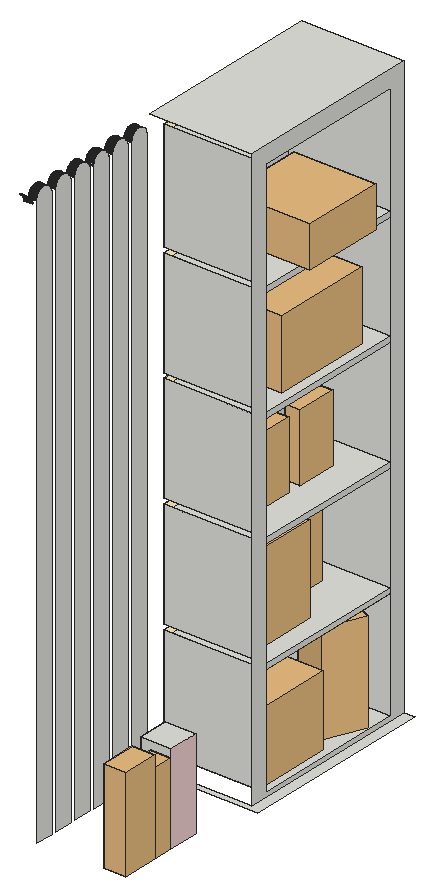
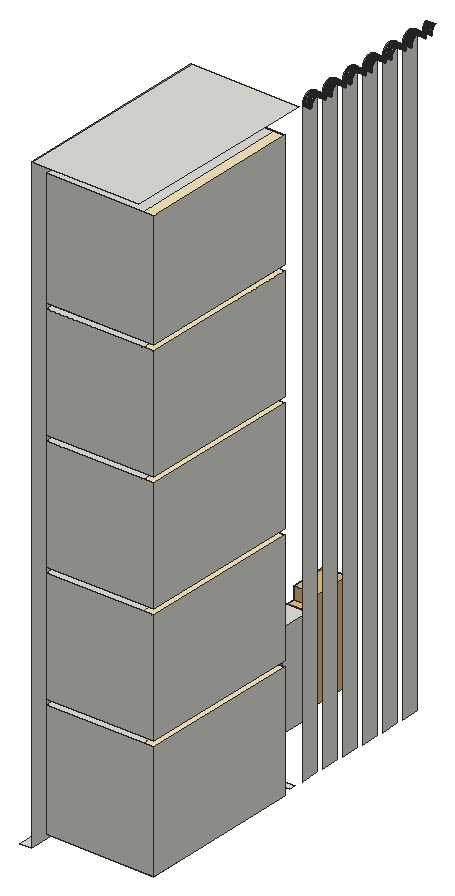
# SketchUp Ruby script. Lengths in inches.
U = 1.inch
M = Sketchup.active_model
def pt(a) = Geom::Point3d.new(a.map { |v| v * U })
def face(e, loops, mat)
  f = e.add_face(loops[0].map { |a| pt(a) })
  loops[1..].each { |l| e.add_face(l.map { |a| pt(a) }).erase! }
  f.material = f.back_material = mat if mat
  f
end
# faces: each face lists its corners as indices into pts; further lists are holes
def faces(e, pts, list, mat = nil) = list.each { |f| face(e, (f[0].is_a?(Array) ? f : [f]).map { |l| l.map { |i| pts[i] } }, mat) }
# xy, xz, yz: faces in a plane at the given z, y or x. An outline is a flat list of corners, or four numbers for a rectangle; further outlines are holes
def ring(l) = l.size == 4 ? [[l[0], l[1]], [l[2], l[1]], [l[2], l[3]], [l[0], l[3]]] : l.each_slice(2).to_a
def flat(e, list, mat, &to3) = list.each { |f| face(e, (f[0].is_a?(Array) ? f : [f]).map { |l| ring(l).map { |u, v| to3.(u, v) } }, mat) }
def xy(e, z, list, mat = nil) = flat(e, list, mat) { |x, y| [x, y, z] }
def xz(e, y, list, mat = nil) = flat(e, list, mat) { |x, z| [x, y, z] }
def yz(e, x, list, mat = nil) = flat(e, list, mat) { |y, z| [x, y, z] }
def lines(e, pts, list) = list.each { |a, b| e.add_line(pt(pts[a]), pt(pts[b])) }
# prism: a flat outline (further loops are holes) pulled along v
def prism(e, loops, v, mat = nil)
  f = face(e, loops, mat); d = Geom::Vector3d.new(v.map { |x| x * U })
  f.pushpull(f.normal.samedirection?(d) ? d.length : -d.length)
end
def box(e, o, s, mat = nil) = prism(e, [[o, [o[0] + s[0], o[1], o[2]], [o[0] + s[0], o[1] + s[1], o[2]], [o[0], o[1] + s[1], o[2]]]], [0, 0, s[2]], mat)
def at(x, y, z, deg = 0) = Geom::Transformation.translation(pt([x, y, z])) * Geom::Transformation.rotation(ORIGIN, Z_AXIS, deg.degrees)
def axes(o, x, y, z) = Geom::Transformation.new([*x, 0, *y, 0, *z, 0, *pt(o).to_a, 1])
def part(name) = M.definitions.add(name)
# library, detail: a bought-in or finely detailed component or shape, given as its bounding box
def library(name, o, s) = part(name).tap { |d| box(d.entities, o, s) }
def detail(e, o, s) = box(e.add_group.entities, o, s)
def put(e, d, t, mat = nil) = e.add_instance(d, t).tap { |i| i.material = mat if mat }
def group(e, t, mat = nil) = e.add_group.tap { |g| g.transformation = t; g.material = mat if mat }.entities
root = M.entities
M.materials.add("Heather_PantShadow").color = [249, 233, 187]
M.materials.add("Pomeli-edt-511x511").color = [242, 209, 211]
M.materials.add("profumo-muschio-natures-511x511").color = [223, 234, 229]
c1 = library("Toiletry bottle \#3",[0,0,0],[4.22,2.62,10.91])
c2 = library("Toiletry bottle \#1",[0,0,0],[3.45,3.45,11.12])
c3 = part("Component\#17")
xy(c3.entities,0,[[0,0,3.21,3.15]],"profumo-muschio-natures-511x511")
xy(c3.entities,9.32,[[0,0,3.21,3.15]])
xz(c3.entities,0,[[0,0,3.21,9.32]],"Pomeli-edt-511x511")
xz(c3.entities,3.15,[[0,0,3.21,9.32]])
yz(c3.entities,0,[[0,0,3.15,9.32]])
yz(c3.entities,3.21,[[0,0,3.15,9.32]])
c4 = library("FILE+KEEPER",[308.125,87.4375,-0.08],[14,9.09,13.53])
c5 = library("Group\#6",[0,0,0],[23.16,7,38.98])
c6 = library("Plant",[-15.17,-14.95,0],[35.27,31.45,46.14])
c7 = library("ADORNOS+-+RMLLR",[6.19,-1.3125,-0.22],[15.35,11.9,12.07])
c8 = library("Potted plant",[0.24,-1.94,0],[14.49,14.49,6.23])
c9 = library("Group\#5",[0,0,0],[23.16,7,38.98])
c10 = library("Man+sculpture",[-5.14,-9.4,0],[7.87,19.56,27.58])
c11 = library("Abstract sculpture",[0,0.06,0],[4.875,4.76,11.74])
xy(root,39.466,[[10,88.07,22.25,88.07,22.25,111,21,111,21,88.732,10,88.732]])
xy(root,40,[[9,90.732,21,109]])
xy(root,52.9,[[10.106,90.732,21,108.993],[9,108.993,21,109]])
xy(root,52.9,[[9,90.732,10.106,108.993]],"Heather_PantShadow")
xy(root,53.5,[[9,90.732,21,109]])
xy(root,66.1,[[10.106,90.732,21,108.993],[9,108.993,21,109]])
xy(root,66.1,[[9,90.732,10.106,108.993]],"Heather_PantShadow")
xy(root,66.7,[[9,90.732,21,109]])
xy(root,79.3,[[10.106,90.732,21,108.993],[9,108.993,10.106,109],[10.106,108.993,21,109]])
xy(root,79.3,[[9,90.732,10.106,108.993]],"Heather_PantShadow")
xy(root,79.9,[[9,90.732,21,109]])
xy(root,92.5,[[10.106,90.732,21,108.993],[9,108.993,10.106,109],[10.106,108.993,21,109]])
xy(root,92.5,[[9,90.732,10.106,108.993]],"Heather_PantShadow")
xy(root,93.1,[[9,90.732,21,109]])
xy(root,106,[[10.106,90.732,21,109]])
xy(root,106,[[9,90.732,10.106,109]],"Heather_PantShadow")
xy(root,108,[[9,71.967,10,72.076],[9,74.755,10,74.864],[9,77.542,10,77.651],[9,80.33,10,80.439],[9,83.117,10,83.226],
  [9,85.905,10,86.014],[9,88.732,21,111]])
xz(root,90.732,[[9,40,21,52.9],[9,53.5,21,66.1],[9,66.7,21,79.3],[9,79.9,21,92.5],[9,93.1,21,106]])
xz(root,109,[[9,40,21,52.9],[9,53.5,21,66.1],[9,66.7,21,79.3],[9,79.9,21,92.5],[9,93.1,21,106]])
yz(root,9,[[90.732,40,109,52.9],[90.732,53.5,109,66.1],[90.732,66.7,109,79.3],[90.732,79.9,109,92.5],[90.732,93.1,109,106],
  [71.967,108,72.076,108,72.022,108.001],[74.755,108,74.864,108,74.809,108.001],[77.542,108,77.651,108,77.597,108.001],[80.33,108,80.439,108,80.384,108.001],[83.117,108,83.226,108,83.172,108.001],
  [85.905,108,86.014,108,85.959,108.001]])
yz(root,10,[[70.981,39.466,73.0625,39.466,73.0625,106.961,73.061,107.015,73.057,107.069,73.05,107.123,73.04,107.177,73.027,107.23,73.012,107.282,72.993,107.334,72.973,107.384,72.949,107.433,72.923,107.481,72.895,107.528,72.864,107.572,72.831,107.616,72.795,107.657,72.758,107.697,72.718,107.734,72.677,107.769,72.633,107.803,72.589,107.834,72.542,107.862,72.494,107.888,72.445,107.911,72.395,107.932,72.343,107.95,72.291,107.966,72.238,107.979,72.185,107.989,72.131,107.996,72.076,108,71.967,108,71.913,107.996,71.859,107.989,71.805,107.979,71.752,107.966,71.7,107.95,71.649,107.932,71.598,107.911,71.549,107.888,71.501,107.862,71.455,107.834,71.41,107.803,71.367,107.769,71.325,107.734,71.286,107.697,71.248,107.657,71.213,107.616,71.18,107.572,71.149,107.528,71.12,107.481,71.094,107.433,71.071,107.384,71.05,107.334,71.032,107.282,71.016,107.23,71.004,107.177,70.994,107.123,70.987,107.069,70.982,107.015,70.981,106.961],[73.768,39.466,75.85,39.466,75.85,106.961,75.849,107.015,75.844,107.069,75.837,107.123,75.827,107.177,75.815,107.23,75.799,107.282,75.781,107.334,75.76,107.384,75.737,107.433,75.711,107.481,75.682,107.528,75.651,107.572,75.618,107.616,75.583,107.657,75.545,107.697,75.506,107.734,75.464,107.769,75.421,107.803,75.376,107.834,75.33,107.862,75.282,107.888,75.233,107.911,75.182,107.932,75.131,107.95,75.079,107.966,75.026,107.979,74.972,107.989,74.918,107.996,74.864,108,74.755,108,74.7,107.996,74.646,107.989,74.593,107.979,74.54,107.966,74.488,107.95,74.436,107.932,74.386,107.911,74.337,107.888,74.289,107.862,74.242,107.834,74.198,107.803,74.154,107.769,74.113,107.734,74.073,107.697,74.036,107.657,74,107.616,73.967,107.572,73.936,107.528,73.908,107.481,73.882,107.433,73.858,107.384,73.838,107.334,73.819,107.282,73.804,107.23,73.791,107.177,73.781,107.123,73.774,107.069,73.77,107.015,73.768,106.961],[76.556,39.466,78.637,39.466,78.637,106.961,78.636,107.015,78.632,107.069,78.625,107.123,78.615,107.177,78.602,107.23,78.587,107.282,78.568,107.334,78.548,107.384,78.524,107.433,78.498,107.481,78.47,107.528,78.439,107.572,78.406,107.616,78.37,107.657,78.333,107.697,78.293,107.734,78.252,107.769,78.208,107.803,78.164,107.834,78.117,107.862,78.069,107.888,78.02,107.911,77.97,107.932,77.918,107.95,77.866,107.966,77.813,107.979,77.76,107.989,77.706,107.996,77.651,108,77.542,108,77.488,107.996,77.434,107.989,77.38,107.979,77.327,107.966,77.275,107.95,77.224,107.932,77.173,107.911,77.124,107.888,77.076,107.862,77.03,107.834,76.985,107.803,76.942,107.769,76.9,107.734,76.861,107.697,76.823,107.657,76.788,107.616,76.755,107.572,76.724,107.528,76.695,107.481,76.669,107.433,76.646,107.384,76.625,107.334,76.607,107.282,76.591,107.23,76.579,107.177,76.569,107.123,76.562,107.069,76.557,107.015,76.556,106.961],[79.343,39.466,81.425,39.466,81.425,106.961,81.424,107.015,81.419,107.069,81.412,107.123,81.402,107.177,81.39,107.23,81.374,107.282,81.356,107.334,81.335,107.384,81.312,107.433,81.286,107.481,81.257,107.528,81.226,107.572,81.193,107.616,81.158,107.657,81.12,107.697,81.081,107.734,81.039,107.769,80.996,107.803,80.951,107.834,80.905,107.862,80.857,107.888,80.808,107.911,80.757,107.932,80.706,107.95,80.654,107.966,80.601,107.979,80.547,107.989,80.493,107.996,80.439,108,80.33,108,80.275,107.996,80.221,107.989,80.168,107.979,80.115,107.966,80.0625,107.95,80.011,107.932,79.961,107.911,79.912,107.888,79.864,107.862,79.817,107.834,79.773,107.803,79.729,107.769,79.688,107.734,79.648,107.697,79.611,107.657,79.575,107.616,79.542,107.572,79.511,107.528,79.483,107.481,79.457,107.433,79.433,107.384,79.413,107.334,79.394,107.282,79.379,107.23,79.366,107.177,79.356,107.123,79.349,107.069,79.345,107.015,79.343,106.961],[82.131,39.466,84.212,39.466,84.212,106.961,84.211,107.015,84.207,107.069,84.2,107.123,84.19,107.177,84.177,107.23,84.162,107.282,84.143,107.334,84.123,107.384,84.099,107.433,84.073,107.481,84.045,107.528,84.014,107.572,83.981,107.616,83.945,107.657,83.908,107.697,83.868,107.734,83.827,107.769,83.783,107.803,83.739,107.834,83.692,107.862,83.644,107.888,83.595,107.911,83.545,107.932,83.493,107.95,83.441,107.966,83.388,107.979,83.335,107.989,83.281,107.996,83.226,108,83.117,108,83.063,107.996,83.009,107.989,82.955,107.979,82.902,107.966,82.85,107.95,82.799,107.932,82.748,107.911,82.699,107.888,82.651,107.862,82.605,107.834,82.56,107.803,82.517,107.769,82.475,107.734,82.436,107.697,82.398,107.657,82.363,107.616,82.33,107.572,82.299,107.528,82.27,107.481,82.244,107.433,82.221,107.384,82.2,107.334,82.182,107.282,82.166,107.23,82.154,107.177,82.144,107.123,82.137,107.069,82.132,107.015,82.131,106.961],
  [84.918,39.466,87,39.466,87,106.961,86.999,107.015,86.994,107.069,86.987,107.123,86.977,107.177,86.965,107.23,86.949,107.282,86.931,107.334,86.91,107.384,86.887,107.433,86.861,107.481,86.832,107.528,86.801,107.572,86.768,107.616,86.733,107.657,86.695,107.697,86.656,107.734,86.614,107.769,86.571,107.803,86.526,107.834,86.48,107.862,86.432,107.888,86.383,107.911,86.332,107.932,86.281,107.95,86.229,107.966,86.176,107.979,86.122,107.989,86.068,107.996,86.014,108,85.905,108,85.85,107.996,85.796,107.989,85.743,107.979,85.69,107.966,85.638,107.95,85.586,107.932,85.536,107.911,85.487,107.888,85.439,107.862,85.392,107.834,85.348,107.803,85.304,107.769,85.263,107.734,85.223,107.697,85.186,107.657,85.15,107.616,85.117,107.572,85.086,107.528,85.058,107.481,85.032,107.433,85.008,107.384,84.988,107.334,84.969,107.282,84.954,107.23,84.941,107.177,84.931,107.123,84.924,107.069,84.92,107.015,84.918,106.961]])
yz(root,21,[[[88.732,39.466,111,108],[90.732,40,109,106]],[90.732,52.9,109,53.5],[90.732,66.1,109,66.7],[90.732,79.3,109,79.9],[90.732,92.5,109,93.1]])
p = [[9,70.274,107.015],[9,70.269,107.069],[10,70.269,107.069],[10,70.274,107.015],[9,70.275,106.961],[10,70.275,106.961],
  [9,70.982,107.015],[9,70.981,106.961],[10,70.981,106.961],[10,70.982,107.015],[9,70.987,107.069],[10,70.987,107.069],
  [9,73.061,107.015],[9,73.057,107.069],[10,73.057,107.069],[10,73.061,107.015],[9,73.0625,106.961],[10,73.0625,106.961],
  [9,73.77,107.015],[9,73.768,106.961],[10,73.768,106.961],[10,73.77,107.015],[9,73.774,107.069],[10,73.774,107.069],
  [9,75.849,107.015],[9,75.844,107.069],[10,75.844,107.069],[10,75.849,107.015],[9,75.85,106.961],[10,75.85,106.961],
  [9,76.557,107.015],[9,76.556,106.961],[10,76.556,106.961],[10,76.557,107.015],[9,76.562,107.069],[10,76.562,107.069],
  [9,78.636,107.015],[9,78.632,107.069],[10,78.632,107.069],[10,78.636,107.015],[9,78.637,106.961],[10,78.637,106.961],
  [9,79.345,107.015],[9,79.343,106.961],[10,79.343,106.961],[10,79.345,107.015],[9,79.349,107.069],[10,79.349,107.069],
  [9,81.424,107.015],[9,81.419,107.069],[10,81.419,107.069],[10,81.424,107.015],[9,81.425,106.961],[10,81.425,106.961],
  [9,82.132,107.015],[9,82.131,106.961],[10,82.131,106.961],[10,82.132,107.015],[9,82.137,107.069],[10,82.137,107.069],
  [9,84.211,107.015],[9,84.207,107.069],[10,84.207,107.069],[10,84.211,107.015],[9,84.212,106.961],[10,84.212,106.961],
  [9,84.92,107.015],[9,84.918,106.961],[10,84.918,106.961],[10,84.92,107.015],[9,84.924,107.069],[10,84.924,107.069],
  [9,86.999,107.015],[9,86.994,107.069],[10,86.994,107.069],[10,86.999,107.015],[9,87,106.961],[10,87,106.961],
  [9,70.262,107.123],[9,70.252,107.177],[10,70.252,107.177],[10,70.262,107.123],[9,70.994,107.123],[10,70.994,107.123],
  [9,71.004,107.177],[10,71.004,107.177],[9,73.05,107.123],[9,73.04,107.177],[10,73.04,107.177],[10,73.05,107.123],
  [9,73.781,107.123],[10,73.781,107.123],[9,73.791,107.177],[10,73.791,107.177],[9,75.837,107.123],[9,75.827,107.177],
  [10,75.827,107.177],[10,75.837,107.123],[9,76.569,107.123],[10,76.569,107.123],[9,76.579,107.177],[10,76.579,107.177],
  [9,78.625,107.123],[9,78.615,107.177],[10,78.615,107.177],[10,78.625,107.123],[9,79.356,107.123],[10,79.356,107.123],
  [9,79.366,107.177],[10,79.366,107.177],[9,81.412,107.123],[9,81.402,107.177],[10,81.402,107.177],[10,81.412,107.123],
  [9,82.144,107.123],[10,82.144,107.123],[9,82.154,107.177],[10,82.154,107.177],[9,84.2,107.123],[9,84.19,107.177],
  [10,84.19,107.177],[10,84.2,107.123],[9,84.931,107.123],[10,84.931,107.123],[9,84.941,107.177],[10,84.941,107.177],
  [9,86.987,107.123],[9,86.977,107.177],[10,86.977,107.177],[10,86.987,107.123],[9,70.24,107.23],[9,70.224,107.282],
  [10,70.224,107.282],[10,70.24,107.23],[9,71.016,107.23],[10,71.016,107.23],[9,71.032,107.282],[10,71.032,107.282],
  [9,73.027,107.23],[9,73.012,107.282],[10,73.012,107.282],[10,73.027,107.23],[9,73.804,107.23],[10,73.804,107.23],
  [9,73.819,107.282],[10,73.819,107.282],[9,75.815,107.23],[9,75.799,107.282],[10,75.799,107.282],[10,75.815,107.23],
  [9,76.591,107.23],[10,76.591,107.23],[9,76.607,107.282],[10,76.607,107.282],[9,78.602,107.23],[9,78.587,107.282],
  [10,78.587,107.282],[10,78.602,107.23],[9,79.379,107.23],[10,79.379,107.23],[9,79.394,107.282],[10,79.394,107.282],
  [9,81.39,107.23],[9,81.374,107.282],[10,81.374,107.282],[10,81.39,107.23],[9,82.166,107.23],[10,82.166,107.23],
  [9,82.182,107.282],[10,82.182,107.282],[9,84.177,107.23],[9,84.162,107.282],[10,84.162,107.282],[10,84.177,107.23],
  [9,84.954,107.23],[10,84.954,107.23],[9,84.969,107.282],[10,84.969,107.282],[9,86.965,107.23],[9,86.949,107.282],
  [10,86.949,107.282],[10,86.965,107.23],[9,70.206,107.334],[9,70.185,107.384],[10,70.185,107.384],[10,70.206,107.334],
  [9,71.05,107.334],[10,71.05,107.334],[9,71.071,107.384],[10,71.071,107.384],[9,72.993,107.334],[9,72.973,107.384],
  [10,72.973,107.384],[10,72.993,107.334],[9,73.838,107.334],[10,73.838,107.334],[9,73.858,107.384],[10,73.858,107.384],
  [9,75.781,107.334],[9,75.76,107.384],[10,75.76,107.384],[10,75.781,107.334],[9,76.625,107.334],[10,76.625,107.334],
  [9,76.646,107.384],[10,76.646,107.384],[9,78.568,107.334],[9,78.548,107.384],[10,78.548,107.384],[10,78.568,107.334],
  [9,79.413,107.334],[10,79.413,107.334],[9,79.433,107.384],[10,79.433,107.384],[9,81.356,107.334],[9,81.335,107.384],
  [10,81.335,107.384],[10,81.356,107.334],[9,82.2,107.334],[10,82.2,107.334],[9,82.221,107.384],[10,82.221,107.384],
  [9,84.143,107.334],[9,84.123,107.384],[10,84.123,107.384],[10,84.143,107.334],[9,84.988,107.334],[10,84.988,107.334],
  [9,85.008,107.384],[10,85.008,107.384],[9,86.931,107.334],[9,86.91,107.384],[10,86.91,107.384],[10,86.931,107.334],
  [9,70.162,107.433],[9,70.136,107.481],[10,70.136,107.481],[10,70.162,107.433],[9,71.094,107.433],[10,71.094,107.433],
  [9,71.12,107.481],[10,71.12,107.481],[9,72.949,107.433],[9,72.923,107.481],[10,72.923,107.481],[10,72.949,107.433],
  [9,73.882,107.433],[10,73.882,107.433],[9,73.908,107.481],[10,73.908,107.481],[9,75.737,107.433],[9,75.711,107.481],
  [10,75.711,107.481],[10,75.737,107.433],[9,76.669,107.433],[10,76.669,107.433],[9,76.695,107.481],[10,76.695,107.481],
  [9,78.524,107.433],[9,78.498,107.481],[10,78.498,107.481],[10,78.524,107.433],[9,79.457,107.433],[10,79.457,107.433],
  [9,79.483,107.481],[10,79.483,107.481],[9,81.312,107.433],[9,81.286,107.481],[10,81.286,107.481],[10,81.312,107.433],
  [9,82.244,107.433],[10,82.244,107.433],[9,82.27,107.481],[10,82.27,107.481],[9,84.099,107.433],[9,84.073,107.481],
  [10,84.073,107.481],[10,84.099,107.433],[9,85.032,107.433],[10,85.032,107.433],[9,85.058,107.481],[10,85.058,107.481],
  [9,86.887,107.433],[9,86.861,107.481],[10,86.861,107.481],[10,86.887,107.433],[9,70.107,107.528],[9,70.076,107.572],
  [10,70.076,107.572],[10,70.107,107.528],[9,71.149,107.528],[10,71.149,107.528],[9,71.18,107.572],[10,71.18,107.572],
  [9,72.895,107.528],[9,72.864,107.572],[10,72.864,107.572],[10,72.895,107.528],[9,73.936,107.528],[10,73.936,107.528],
  [9,73.967,107.572],[10,73.967,107.572],[9,75.682,107.528],[9,75.651,107.572],[10,75.651,107.572],[10,75.682,107.528],
  [9,76.724,107.528],[10,76.724,107.528],[9,76.755,107.572],[10,76.755,107.572],[9,78.47,107.528],[9,78.439,107.572],
  [10,78.439,107.572],[10,78.47,107.528],[9,79.511,107.528],[10,79.511,107.528],[9,79.542,107.572],[10,79.542,107.572],
  [9,81.257,107.528],[9,81.226,107.572],[10,81.226,107.572],[10,81.257,107.528],[9,82.299,107.528],[10,82.299,107.528],
  [9,82.33,107.572],[10,82.33,107.572],[9,84.045,107.528],[9,84.014,107.572],[10,84.014,107.572],[10,84.045,107.528],
  [9,85.086,107.528],[10,85.086,107.528],[9,85.117,107.572],[10,85.117,107.572],[9,86.832,107.528],[9,86.801,107.572],
  [10,86.801,107.572],[10,86.832,107.528],[9,70.043,107.616],[9,70.008,107.657],[10,70.008,107.657],[10,70.043,107.616],
  [9,71.213,107.616],[10,71.213,107.616],[9,71.248,107.657],[10,71.248,107.657],[9,72.831,107.616],[9,72.795,107.657],
  [10,72.795,107.657],[10,72.831,107.616],[9,74,107.616],[10,74,107.616],[9,74.036,107.657],[10,74.036,107.657],
  [9,75.618,107.616],[9,75.583,107.657],[10,75.583,107.657],[10,75.618,107.616],[9,76.788,107.616],[10,76.788,107.616],
  [9,76.823,107.657],[10,76.823,107.657],[9,78.406,107.616],[9,78.37,107.657],[10,78.37,107.657],[10,78.406,107.616],
  [9,79.575,107.616],[10,79.575,107.616],[9,79.611,107.657],[10,79.611,107.657],[9,81.193,107.616],[9,81.158,107.657],
  [10,81.158,107.657],[10,81.193,107.616],[9,82.363,107.616],[10,82.363,107.616],[9,82.398,107.657],[10,82.398,107.657],
  [9,83.981,107.616],[9,83.945,107.657],[10,83.945,107.657],[10,83.981,107.616],[9,85.15,107.616],[10,85.15,107.616],
  [9,85.186,107.657],[10,85.186,107.657],[9,86.768,107.616],[9,86.733,107.657],[10,86.733,107.657],[10,86.768,107.616],
  [9,69.931,107.734],[9,69.889,107.769],[10,69.889,107.769],[10,69.931,107.734],[9,69.97,107.697],[10,69.97,107.697],
  [9,71.286,107.697],[10,71.286,107.697],[9,71.325,107.734],[10,71.325,107.734],[9,71.367,107.769],[10,71.367,107.769],
  [9,72.718,107.734],[9,72.677,107.769],[10,72.677,107.769],[10,72.718,107.734],[9,72.758,107.697],[10,72.758,107.697],
  [9,74.073,107.697],[10,74.073,107.697],[9,74.113,107.734],[10,74.113,107.734],[9,74.154,107.769],[10,74.154,107.769],
  [9,75.506,107.734],[9,75.464,107.769],[10,75.464,107.769],[10,75.506,107.734],[9,75.545,107.697],[10,75.545,107.697],
  [9,76.861,107.697],[10,76.861,107.697],[9,76.9,107.734],[10,76.9,107.734],[9,76.942,107.769],[10,76.942,107.769],
  [9,78.293,107.734],[9,78.252,107.769],[10,78.252,107.769],[10,78.293,107.734],[9,78.333,107.697],[10,78.333,107.697],
  [9,79.648,107.697],[10,79.648,107.697],[9,79.688,107.734],[10,79.688,107.734],[9,79.729,107.769],[10,79.729,107.769],
  [9,81.081,107.734],[9,81.039,107.769],[10,81.039,107.769],[10,81.081,107.734],[9,81.12,107.697],[10,81.12,107.697],
  [9,82.436,107.697],[10,82.436,107.697],[9,82.475,107.734],[10,82.475,107.734],[9,82.517,107.769],[10,82.517,107.769],
  [9,83.868,107.734],[9,83.827,107.769],[10,83.827,107.769],[10,83.868,107.734],[9,83.908,107.697],[10,83.908,107.697],
  [9,85.223,107.697],[10,85.223,107.697],[9,85.263,107.734],[10,85.263,107.734],[9,85.304,107.769],[10,85.304,107.769],
  [9,86.656,107.734],[9,86.614,107.769],[10,86.614,107.769],[10,86.656,107.734],[9,86.695,107.697],[10,86.695,107.697],
  [9,69.801,107.834],[9,69.755,107.862],[10,69.755,107.862],[10,69.801,107.834],[9,69.846,107.803],[10,69.846,107.803],
  [9,71.41,107.803],[10,71.41,107.803],[9,71.455,107.834],[10,71.455,107.834],[9,71.501,107.862],[10,71.501,107.862],
  [9,72.589,107.834],[9,72.542,107.862],[10,72.542,107.862],[10,72.589,107.834],[9,72.633,107.803],[10,72.633,107.803],
  [9,74.198,107.803],[10,74.198,107.803],[9,74.242,107.834],[10,74.242,107.834],[9,74.289,107.862],[10,74.289,107.862],
  [9,75.376,107.834],[9,75.33,107.862],[10,75.33,107.862],[10,75.376,107.834],[9,75.421,107.803],[10,75.421,107.803],
  [9,76.985,107.803],[10,76.985,107.803],[9,77.03,107.834],[10,77.03,107.834],[9,77.076,107.862],[10,77.076,107.862],
  [9,78.164,107.834],[9,78.117,107.862],[10,78.117,107.862],[10,78.164,107.834],[9,78.208,107.803],[10,78.208,107.803],
  [9,79.773,107.803],[10,79.773,107.803],[9,79.817,107.834],[10,79.817,107.834],[9,79.864,107.862],[10,79.864,107.862],
  [9,80.951,107.834],[9,80.905,107.862],[10,80.905,107.862],[10,80.951,107.834],[9,80.996,107.803],[10,80.996,107.803],
  [9,82.56,107.803],[10,82.56,107.803],[9,82.605,107.834],[10,82.605,107.834],[9,82.651,107.862],[10,82.651,107.862],
  [9,83.739,107.834],[9,83.692,107.862],[10,83.692,107.862],[10,83.739,107.834],[9,83.783,107.803],[10,83.783,107.803],
  [9,85.348,107.803],[10,85.348,107.803],[9,85.392,107.834],[10,85.392,107.834],[9,85.439,107.862],[10,85.439,107.862],
  [9,86.526,107.834],[9,86.48,107.862],[10,86.48,107.862],[10,86.526,107.834],[9,86.571,107.803],[10,86.571,107.803],
  [9,69.707,107.888],[10,69.707,107.888],[9,71.549,107.888],[10,71.549,107.888],[9,71.598,107.911],[10,71.598,107.911],
  [9,71.649,107.932],[10,71.649,107.932],[9,71.7,107.95],[10,71.7,107.95],[9,72.395,107.932],[9,72.343,107.95],
  [10,72.343,107.95],[10,72.395,107.932],[9,72.445,107.911],[10,72.445,107.911],[9,72.494,107.888],[10,72.494,107.888],
  [9,74.337,107.888],[10,74.337,107.888],[9,74.386,107.911],[10,74.386,107.911],[9,74.436,107.932],[10,74.436,107.932],
  [9,74.488,107.95],[10,74.488,107.95],[9,75.182,107.932],[9,75.131,107.95],[10,75.131,107.95],[10,75.182,107.932],
  [9,75.233,107.911],[10,75.233,107.911],[9,75.282,107.888],[10,75.282,107.888],[9,77.124,107.888],[10,77.124,107.888],
  [9,77.173,107.911],[10,77.173,107.911],[9,77.224,107.932],[10,77.224,107.932],[9,77.275,107.95],[10,77.275,107.95],
  [9,77.97,107.932],[9,77.918,107.95],[10,77.918,107.95],[10,77.97,107.932],[9,78.02,107.911],[10,78.02,107.911],
  [9,78.069,107.888],[10,78.069,107.888],[9,79.912,107.888],[10,79.912,107.888],[9,79.961,107.911],[10,79.961,107.911],
  [9,80.011,107.932],[10,80.011,107.932],[9,80.0625,107.95],[10,80.0625,107.95],[9,80.757,107.932],[9,80.706,107.95],
  [10,80.706,107.95],[10,80.757,107.932],[9,80.808,107.911],[10,80.808,107.911],[9,80.857,107.888],[10,80.857,107.888],
  [9,82.699,107.888],[10,82.699,107.888],[9,82.748,107.911],[10,82.748,107.911],[9,82.799,107.932],[10,82.799,107.932],
  [9,82.85,107.95],[10,82.85,107.95],[9,83.545,107.932],[9,83.493,107.95],[10,83.493,107.95],[10,83.545,107.932],
  [9,83.595,107.911],[10,83.595,107.911],[9,83.644,107.888],[10,83.644,107.888],[9,85.487,107.888],[10,85.487,107.888],
  [9,85.536,107.911],[10,85.536,107.911],[9,85.586,107.932],[10,85.586,107.932],[9,85.638,107.95],[10,85.638,107.95],
  [9,86.332,107.932],[9,86.281,107.95],[10,86.281,107.95],[10,86.332,107.932],[9,86.383,107.911],[10,86.383,107.911],
  [9,86.432,107.888],[10,86.432,107.888],[9,71.752,107.966],[10,71.752,107.966],[9,71.805,107.979],[10,71.805,107.979],
  [9,71.859,107.989],[10,71.859,107.989],[9,71.913,107.996],[10,71.913,107.996],[9,71.967,108],[10,71.967,108],
  [9,72.131,107.996],[9,72.076,108],[10,72.076,108],[10,72.131,107.996],[9,72.185,107.989],[10,72.185,107.989],
  [9,72.238,107.979],[10,72.238,107.979],[9,72.291,107.966],[10,72.291,107.966],[9,74.54,107.966],[10,74.54,107.966],
  [9,74.593,107.979],[10,74.593,107.979],[9,74.646,107.989],[10,74.646,107.989],[9,74.7,107.996],[10,74.7,107.996],
  [9,74.755,108],[10,74.755,108],[9,74.918,107.996],[9,74.864,108],[10,74.864,108],[10,74.918,107.996],
  [9,74.972,107.989],[10,74.972,107.989],[9,75.026,107.979],[10,75.026,107.979],[9,75.079,107.966],[10,75.079,107.966],
  [9,77.327,107.966],[10,77.327,107.966],[9,77.38,107.979],[10,77.38,107.979],[9,77.434,107.989],[10,77.434,107.989],
  [9,77.488,107.996],[10,77.488,107.996],[9,77.542,108],[10,77.542,108],[9,77.706,107.996],[9,77.651,108],
  [10,77.651,108],[10,77.706,107.996],[9,77.76,107.989],[10,77.76,107.989],[9,77.813,107.979],[10,77.813,107.979],
  [9,77.866,107.966],[10,77.866,107.966],[9,80.115,107.966],[10,80.115,107.966],[9,80.168,107.979],[10,80.168,107.979],
  [9,80.221,107.989],[10,80.221,107.989],[9,80.275,107.996],[10,80.275,107.996],[9,80.33,108],[10,80.33,108],
  [9,80.493,107.996],[9,80.439,108],[10,80.439,108],[10,80.493,107.996],[9,80.547,107.989],[10,80.547,107.989],
  [9,80.601,107.979],[10,80.601,107.979],[9,80.654,107.966],[10,80.654,107.966],[9,82.902,107.966],[10,82.902,107.966],
  [9,82.955,107.979],[10,82.955,107.979],[9,83.009,107.989],[10,83.009,107.989],[9,83.063,107.996],[10,83.063,107.996],
  [9,83.117,108],[10,83.117,108],[9,83.281,107.996],[9,83.226,108],[10,83.226,108],[10,83.281,107.996],
  [9,83.335,107.989],[10,83.335,107.989],[9,83.388,107.979],[10,83.388,107.979],[9,83.441,107.966],[10,83.441,107.966],
  [9,85.69,107.966],[10,85.69,107.966],[9,85.743,107.979],[10,85.743,107.979],[9,85.796,107.989],[10,85.796,107.989],
  [9,85.85,107.996],[10,85.85,107.996],[9,85.905,108],[10,85.905,108],[9,86.068,107.996],[9,86.014,108],
  [10,86.014,108],[10,86.068,107.996],[9,86.122,107.989],[10,86.122,107.989],[9,86.176,107.979],[10,86.176,107.979],
  [9,86.229,107.966],[10,86.229,107.966],[9,90.725,52.9],[9,90.732,52.9],[9,90.725,92.5],[9,90.732,92.5],
  [9,90.725,66.1],[9,90.732,66.1],[9,90.725,79.3],[9,90.732,79.3]]
faces(root,p,[[0,1,2,3],[4,0,3,5],[6,7,8,9],[10,6,9,11],[12,13,14,15],[16,12,15,17],[18,19,20,21],[22,18,21,23],
  [24,25,26,27],[28,24,27,29],[30,31,32,33],[34,30,33,35],[36,37,38,39],[40,36,39,41],[42,43,44,45],[46,42,45,47],
  [48,49,50,51],[52,48,51,53],[54,55,56,57],[58,54,57,59],[60,61,62,63],[64,60,63,65],[66,67,68,69],[70,66,69,71],
  [72,73,74,75],[76,72,75,77],[78,79,80,81],[1,78,81,2],[82,10,11,83],[84,82,83,85],[86,87,88,89],[13,86,89,14],
  [90,22,23,91],[92,90,91,93],[94,95,96,97],[25,94,97,26],[98,34,35,99],[100,98,99,101],[102,103,104,105],[37,102,105,38],
  [106,46,47,107],[108,106,107,109],[110,111,112,113],[49,110,113,50],[114,58,59,115],[116,114,115,117],[118,119,120,121],[61,118,121,62],
  [122,70,71,123],[124,122,123,125],[126,127,128,129],[73,126,129,74],[130,131,132,133],[79,130,133,80],[134,84,85,135],[136,134,135,137],
  [138,139,140,141],[87,138,141,88],[142,92,93,143],[144,142,143,145],[146,147,148,149],[95,146,149,96],[150,100,101,151],[152,150,151,153],
  [154,155,156,157],[103,154,157,104],[158,108,109,159],[160,158,159,161],[162,163,164,165],[111,162,165,112],[166,116,117,167],[168,166,167,169],
  [170,171,172,173],[119,170,173,120],[174,124,125,175],[176,174,175,177],[178,179,180,181],[127,178,181,128],[182,183,184,185],[131,182,185,132],
  [186,136,137,187],[188,186,187,189],[190,191,192,193],[139,190,193,140],[194,144,145,195],[196,194,195,197],[198,199,200,201],[147,198,201,148],
  [202,152,153,203],[204,202,203,205],[206,207,208,209],[155,206,209,156],[210,160,161,211],[212,210,211,213],[214,215,216,217],[163,214,217,164],
  [218,168,169,219],[220,218,219,221],[222,223,224,225],[171,222,225,172],[226,176,177,227],[228,226,227,229],[230,231,232,233],[179,230,233,180],
  [234,235,236,237],[183,234,237,184],[238,188,189,239],[240,238,239,241],[242,243,244,245],[191,242,245,192],[246,196,197,247],[248,246,247,249],
  [250,251,252,253],[199,250,253,200],[254,204,205,255],[256,254,255,257],[258,259,260,261],[207,258,261,208],[262,212,213,263],[264,262,263,265],
  [266,267,268,269],[215,266,269,216],[270,220,221,271],[272,270,271,273],[274,275,276,277],[223,274,277,224],[278,228,229,279],[280,278,279,281],
  [282,283,284,285],[231,282,285,232],[286,287,288,289],[235,286,289,236],[290,240,241,291],[292,290,291,293],[294,295,296,297],[243,294,297,244],
  [298,248,249,299],[300,298,299,301],[302,303,304,305],[251,302,305,252],[306,256,257,307],[308,306,307,309],[310,311,312,313],[259,310,313,260],
  [314,264,265,315],[316,314,315,317],[318,319,320,321],[267,318,321,268],[322,272,273,323],[324,322,323,325],[326,327,328,329],[275,326,329,276],
  [330,280,281,331],[332,330,331,333],[334,335,336,337],[283,334,337,284],[338,339,340,341],[287,338,341,288],[342,292,293,343],[344,342,343,345],
  [346,347,348,349],[295,346,349,296],[350,300,301,351],[352,350,351,353],[354,355,356,357],[303,354,357,304],[358,308,309,359],[360,358,359,361],
  [362,363,364,365],[311,362,365,312],[366,316,317,367],[368,366,367,369],[370,371,372,373],[319,370,373,320],[374,324,325,375],[376,374,375,377],
  [378,379,380,381],[327,378,381,328],[382,332,333,383],[384,382,383,385],[386,387,388,389],[335,386,389,336],[390,391,392,393],[394,390,393,395],
  [339,394,395,340],[396,344,345,397],[398,396,397,399],[400,398,399,401],[402,403,404,405],[406,402,405,407],[347,406,407,348],[408,352,353,409],
  [410,408,409,411],[412,410,411,413],[414,415,416,417],[418,414,417,419],[355,418,419,356],[420,360,361,421],[422,420,421,423],[424,422,423,425],
  [426,427,428,429],[430,426,429,431],[363,430,431,364],[432,368,369,433],[434,432,433,435],[436,434,435,437],[438,439,440,441],[442,438,441,443],
  [371,442,443,372],[444,376,377,445],[446,444,445,447],[448,446,447,449],[450,451,452,453],[454,450,453,455],[379,454,455,380],[456,384,385,457],
  [458,456,457,459],[460,458,459,461],[462,463,464,465],[466,462,465,467],[387,466,467,388],[468,469,470,471],[472,468,471,473],[391,472,473,392],
  [474,400,401,475],[476,474,475,477],[478,476,477,479],[480,481,482,483],[484,480,483,485],[403,484,485,404],[486,412,413,487],[488,486,487,489],
  [490,488,489,491],[492,493,494,495],[496,492,495,497],[415,496,497,416],[498,424,425,499],[500,498,499,501],[502,500,501,503],[504,505,506,507],
  [508,504,507,509],[427,508,509,428],[510,436,437,511],[512,510,511,513],[514,512,513,515],[516,517,518,519],[520,516,519,521],[439,520,521,440],
  [522,448,449,523],[524,522,523,525],[526,524,525,527],[528,529,530,531],[532,528,531,533],[451,532,533,452],[534,460,461,535],[536,534,535,537],
  [538,536,537,539],[540,541,542,543],[544,540,543,545],[463,544,545,464],[469,546,547,470],[548,478,479,549],[550,548,549,551],[552,550,551,553],
  [554,552,553,555],[556,557,558,559],[560,556,559,561],[562,560,561,563],[481,562,563,482],[564,490,491,565],[566,564,565,567],[568,566,567,569],
  [570,568,569,571],[572,573,574,575],[576,572,575,577],[578,576,577,579],[493,578,579,494],[580,502,503,581],[582,580,581,583],[584,582,583,585],
  [586,584,585,587],[588,589,590,591],[592,588,591,593],[594,592,593,595],[505,594,595,506],[596,514,515,597],[598,596,597,599],[600,598,599,601],
  [602,600,601,603],[604,605,606,607],[608,604,607,609],[610,608,609,611],[517,610,611,518],[612,526,527,613],[614,612,613,615],[616,614,615,617],
  [618,616,617,619],[620,621,622,623],[624,620,623,625],[626,624,625,627],[529,626,627,530],[628,538,539,629],[630,628,629,631],[632,630,631,633],
  [634,632,633,635],[636,637,638,639],[640,636,639,641],[642,640,641,643],[541,642,643,542],[644,554,555,645],[646,644,645,647],[648,646,647,649],
  [650,648,649,651],[652,650,651,653],[654,655,656,657],[658,654,657,659],[660,658,659,661],[662,660,661,663],[557,662,663,558],[664,570,571,665],
  [666,664,665,667],[668,666,667,669],[670,668,669,671],[672,670,671,673],[674,675,676,677],[678,674,677,679],[680,678,679,681],[682,680,681,683],
  [573,682,683,574],[684,586,587,685],[686,684,685,687],[688,686,687,689],[690,688,689,691],[692,690,691,693],[694,695,696,697],[698,694,697,699],
  [700,698,699,701],[702,700,701,703],[589,702,703,590],[704,602,603,705],[706,704,705,707],[708,706,707,709],[710,708,709,711],[712,710,711,713],
  [714,715,716,717],[718,714,717,719],[720,718,719,721],[722,720,721,723],[605,722,723,606],[724,618,619,725],[726,724,725,727],[728,726,727,729],
  [730,728,729,731],[732,730,731,733],[734,735,736,737],[738,734,737,739],[740,738,739,741],[742,740,741,743],[621,742,743,622],[744,634,635,745],
  [746,744,745,747],[748,746,747,749],[750,748,749,751],[752,750,751,753],[754,755,756,757],[758,754,757,759],[760,758,759,761],[762,760,761,763],
  [637,762,763,638]])
lines(root,p,[[764,765],[766,767],[768,769],[770,771]])
put(root,c1,at(20.1875,71.22,39.47,90))
put(root,c2,axes([20.1875,75.4375,39.47],[0,0.69,0],[-0.69,0,0],[0,0,0.85643]))
put(root,c3,axes([20.1875,77.82,39.47],[0,1.13,0],[-1.13,0,0],[0,0,1.13]))
put(root,c4,axes([-39.39,290.18,40.01],[0,-0.61622,0],[0.61622,0,0],[0,0,0.61622]))
put(root,c5,axes([17.25,94.01,66.57],[0,0.20584,0],[-0.25731,0,0],[0,0,0.20584]))
put(root,c6,axes([14.3,96.27,53.5],[0.22445,0,0],[0,0.22445,0],[0,0,0.22445]))
put(root,c7,axes([19.38,89.3,80.39],[0,0.76608,0],[-0.672,0,0],[0,0,0.672]))
put(root,c8,axes([12.39,97.06,93.1],[0.66461,0,0],[0,0.66461,0],[0,0,0.77354]))
put(root,c9,axes([17.25,100.44,66.57],[0,0.20584,0],[-0.25731,0,0],[0,0,0.20584]))
put(root,c10,axes([14.47,102.92,53.5],[0.31,0,0],[0,0.31,0],[0,0,0.31]))
put(root,c11,at(14.41,103.55,40,-23.8))
